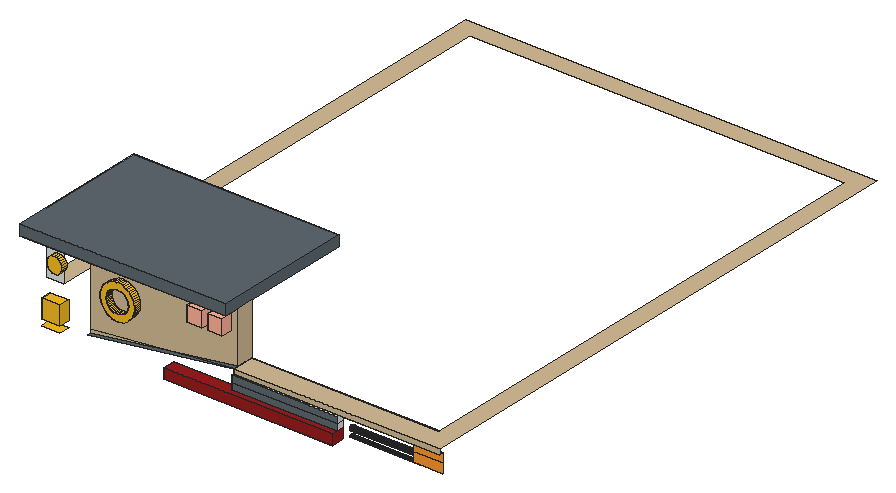
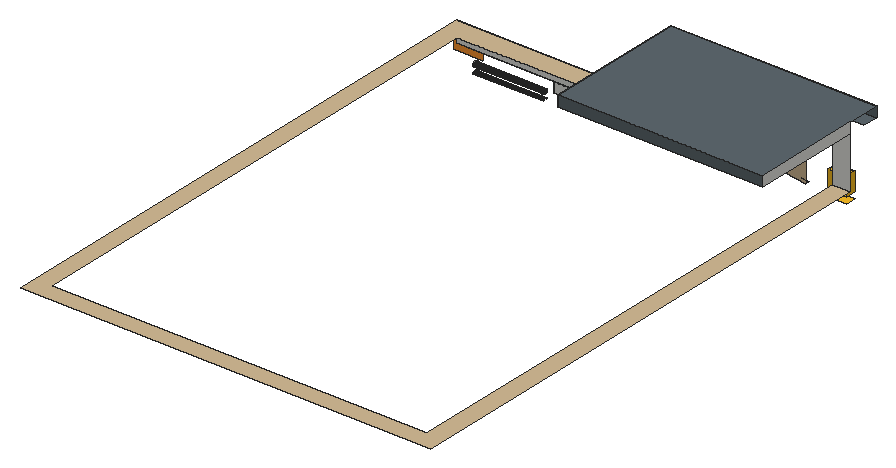
# SketchUp Ruby script. Lengths in inches.
U = 1.inch
M = Sketchup.active_model
def pt(a) = Geom::Point3d.new(a.map { |v| v * U })
def face(e, loops, mat)
  f = e.add_face(loops[0].map { |a| pt(a) })
  loops[1..].each { |l| e.add_face(l.map { |a| pt(a) }).erase! }
  f.material = f.back_material = mat if mat
  f
end
# faces: each face lists its corners as indices into pts; further lists are holes
def faces(e, pts, list, mat = nil) = list.each { |f| face(e, (f[0].is_a?(Array) ? f : [f]).map { |l| l.map { |i| pts[i] } }, mat) }
# xy, xz, yz: faces in a plane at the given z, y or x. An outline is a flat list of corners, or four numbers for a rectangle; further outlines are holes
def ring(l) = l.size == 4 ? [[l[0], l[1]], [l[2], l[1]], [l[2], l[3]], [l[0], l[3]]] : l.each_slice(2).to_a
def flat(e, list, mat, &to3) = list.each { |f| face(e, (f[0].is_a?(Array) ? f : [f]).map { |l| ring(l).map { |u, v| to3.(u, v) } }, mat) }
def xy(e, z, list, mat = nil) = flat(e, list, mat) { |x, y| [x, y, z] }
def xz(e, y, list, mat = nil) = flat(e, list, mat) { |x, z| [x, y, z] }
def yz(e, x, list, mat = nil) = flat(e, list, mat) { |y, z| [x, y, z] }
def lines(e, pts, list) = list.each { |a, b| e.add_line(pt(pts[a]), pt(pts[b])) }
# prism: a flat outline (further loops are holes) pulled along v
def prism(e, loops, v, mat = nil)
  f = face(e, loops, mat); d = Geom::Vector3d.new(v.map { |x| x * U })
  f.pushpull(f.normal.samedirection?(d) ? d.length : -d.length)
end
def box(e, o, s, mat = nil) = prism(e, [[o, [o[0] + s[0], o[1], o[2]], [o[0] + s[0], o[1] + s[1], o[2]], [o[0], o[1] + s[1], o[2]]]], [0, 0, s[2]], mat)
def at(x, y, z, deg = 0) = Geom::Transformation.translation(pt([x, y, z])) * Geom::Transformation.rotation(ORIGIN, Z_AXIS, deg.degrees)
def axes(o, x, y, z) = Geom::Transformation.new([*x, 0, *y, 0, *z, 0, *pt(o).to_a, 1])
def part(name) = M.definitions.add(name)
# library, detail: a bought-in or finely detailed component or shape, given as its bounding box
def library(name, o, s) = part(name).tap { |d| box(d.entities, o, s) }
def detail(e, o, s) = box(e.add_group.entities, o, s)
def put(e, d, t, mat = nil) = e.add_instance(d, t).tap { |i| i.material = mat if mat }
def group(e, t, mat = nil) = e.add_group.tap { |g| g.transformation = t; g.material = mat if mat }.entities
root = M.entities
M.materials.add("[0045_Goldenrod]").color = [249, 189, 36]
M.materials.add("[Color A04]").color = [155, 30, 30]
M.materials.add("[Color B02]").color = [255, 178, 153]
M.materials.add("[Color C04]").color = [255, 153, 50]
M.materials.add("[Formica Beige]").color = [211, 187, 149]
M.materials.add("[Formica Laminate Dark]").color = [50, 53, 60]
M.materials.add("[Formica Speckled Grey]").color = [94, 105, 111]
xy(root,310.29,[[175.33,79.24,383.64,94.74]],"[Color A04]")
xy(root,314.74,[[23.1,81.43,45.78,94.74]],"[0045_Goldenrod]")
xy(root,317.54,[[411.92,104.06,412.58,104.14,413.2,104.4,413.49,104.62,410.35,104.62,410.64,104.4,411.25,104.14],[410.35,104.62,413.49,104.62,413.73,104.81,414.14,105.34,414.39,105.95,414.48,106.62,414.39,107.28,414.14,107.9,413.73,108.43,413.2,108.84,412.58,109.09,411.92,109.18,411.25,109.09,410.64,108.84,410.11,108.43,409.7,107.9,409.44,107.28,409.36,106.62,409.44,105.95,409.7,105.34,410.11,104.81]])
xy(root,318.0625,[[440.11,104.06,440.77,104.14,441.39,104.4,441.92,104.81,442.32,105.34,442.58,105.95,442.67,106.62,442.58,107.28,442.32,107.9,441.92,108.43,441.39,108.84,440.77,109.09,440.11,109.18,439.44,109.09,438.82,108.84,438.29,108.43,437.89,107.9,437.63,107.28,437.54,106.62,437.63,105.95,437.89,105.34,438.29,104.81,438.82,104.4,439.44,104.14]])
xy(root,322.3,[[23.1,81.43,45.78,94.74]],"[0045_Goldenrod]")
xy(root,322.92,[[253.89,86.55,383.64,94.74]])
xy(root,322.92,[[175.33,79.24,383.64,79.24,383.64,86.55,253.89,86.55,253.89,94.74,175.33,94.74]],"[Color A04]")
xy(root,330.28,[[253.89,86.55,383.64,94.74]])
xy(root,338.91,[[253.89,86.55,383.64,89.43],[253.89,89.43,383.64,94.74],[253.89,94.74,383.64,116.19]])
xy(root,338.91,[[383.64,89.43,470.23,116.19],[470.23,89.43,506.36,94.74]],"[Formica Beige]")
xy(root,344.99,[[23.1,81.43,45.78,94.74]],"[0045_Goldenrod]")
xy(root,345.125,[[253.89,89.43,506.36,89.43,506.36,761.28,1.43,761.28,1.43,116.19,22.875,116.19,22.875,739.83,484.91,739.83,484.91,116.19,253.89,116.19]],"[Formica Beige]")
xy(root,381.62,[[202.13,81.55,220.38,94.74],[227.32,81.55,245.57,94.74]],"[Color B02]")
xy(root,399.87,[[202.13,81.55,220.38,94.74],[227.32,81.55,245.57,94.74]],"[Color B02]")
xy(root,408.81,[[1.43,76.18,73.65,94.74],[73.65,76.18,253.89,94.74],[1.43,116.19,253.89,250.25]],"[Formica Speckled Grey]")
xy(root,421.875,[[1.43,76.18,253.89,250.25]],"[Formica Speckled Grey]")
xz(root,76.18,[[1.43,408.81,253.89,421.875]],"[Formica Speckled Grey]")
xz(root,79.24,[[175.33,310.29,383.64,322.92]],"[Color A04]")
xz(root,81.43,[[23.1,322.3,45.78,344.99]],"[0045_Goldenrod]")
xz(root,81.55,[[202.13,381.62,220.38,399.87],[227.32,381.62,245.57,399.87]],"[Color B02]")
xz(root,85.93,[[[113.16,349,115.38,349.14,117.58,349.52,119.73,350.13,121.8,350.95,123.77,351.99,125.63,353.23,127.34,354.66,128.9,356.26,130.28,358.01,131.47,359.9,132.46,361.9,133.23,363.99,133.78,366.15,134.1,368.36,134.18,370.59,134.04,372.82,133.66,375.01,133.05,377.16,132.23,379.23,131.1875,381.21,129.95,383.0625,128.52,384.78,126.92,386.33,125.17,387.71,123.28,388.9,121.28,389.89,119.19,390.66,117.03,391.21,114.82,391.53,112.59,391.62,110.36,391.47,108.17,391.09,106.02,390.49,103.95,389.66,101.97,388.62,100.12,387.38,98.4,385.96,96.85,384.36,95.47,382.61,94.28,380.72,93.29,378.72,92.52,376.625,91.97,374.46,91.65,372.25,91.5625,370.03,91.71,367.8,92.09,365.6,92.69,363.45,93.52,361.38,94.56,359.41,95.8,357.55,97.23,355.84,98.82,354.28,100.58,352.9,102.46,351.71,104.46,350.72,106.56,349.95,108.72,349.4,110.93,349.08],[113.05,356.63,111.625,356.69,110.21,356.89,108.82,357.25,107.48,357.74,106.19,358.375,104.98,359.14,103.86,360.02,102.83,361.02,101.92,362.125,101.12,363.3125,100.46,364.58,99.92,365.91,99.54,367.29,99.29,368.7,99.2,370.125,99.26,371.56,99.46,372.97,99.8125,374.36,100.31,375.7,100.94,376.99,101.7,378.2,102.59,379.32,103.59,380.35,104.6875,381.26,105.88,382.06,107.15,382.73,108.48,383.26,109.85,383.65,111.26,383.89,112.69,383.98,114.12,383.93,115.54,383.72,116.93,383.37,118.27,382.875,119.55,382.24,120.76,381.48,121.89,380.59,122.91,379.59,123.83,378.49,124.625,377.3,125.29,376.03,125.82,374.71,126.21,373.33,126.45,371.92,126.55,370.49,126.49,369.06,126.29,367.64,125.93,366.25,125.4375,364.91,124.81,363.63,124.04,362.42,123.16,361.29,122.16,360.27,121.06,359.35,119.87,358.56,118.6,357.89,117.27,357.36,115.89,356.97,114.48,356.73]]],"[0045_Goldenrod]")
xz(root,86.55,[[253.89,322.92,383.64,330.28],[253.89,330.28,383.64,338.91]],"[Formica Speckled Grey]")
xz(root,87.62,[[34.11,372.72,36.6,373.05,38.92,374.01,40.92,375.54,42.45,377.53,43.41,379.85,43.74,382.34,43.41,384.83,42.45,387.15,40.92,389.15,38.92,390.68,36.6,391.64,34.11,391.97,31.62,391.64,29.3,390.68,27.3,389.15,25.78,387.15,24.8125,384.83,24.49,382.34,24.8125,379.85,25.78,377.53,27.3,375.54,29.3,374.01,31.62,373.05]],"[0045_Goldenrod]")
xz(root,89.43,[[253.89,338.91,506.36,345.125]],"[Formica Beige]")
xz(root,94.74,[[175.33,310.29,383.64,322.92],[253.89,322.92,383.64,330.28],[253.89,330.28,383.64,338.91],[202.13,381.62,220.38,399.87],[227.32,381.62,245.57,399.87]])
xz(root,94.74,[[470.23,315.65,506.36,327.28],[470.23,327.28,506.36,338.91]],"[Color C04]")
xz(root,94.74,[[[73.65,318.75,253.89,345.125,253.89,408.81,73.65,408.81],[113.16,349,110.93,349.08,108.72,349.4,106.56,349.95,104.46,350.72,102.46,351.71,100.58,352.9,98.82,354.28,97.23,355.84,95.8,357.55,94.56,359.41,93.52,361.38,92.69,363.45,92.09,365.6,91.71,367.8,91.5625,370.03,91.65,372.25,91.97,374.46,92.52,376.625,93.29,378.72,94.28,380.72,95.47,382.61,96.85,384.36,98.4,385.96,100.12,387.38,101.97,388.62,103.95,389.66,106.02,390.49,108.17,391.09,110.36,391.47,112.59,391.62,114.82,391.53,117.03,391.21,119.19,390.66,121.28,389.89,123.28,388.9,125.17,387.71,126.92,386.33,128.52,384.78,129.95,383.0625,131.1875,381.21,132.23,379.23,133.05,377.16,133.66,375.01,134.04,372.82,134.18,370.59,134.1,368.36,133.78,366.15,133.23,363.99,132.46,361.9,131.47,359.9,130.28,358.01,128.9,356.26,127.34,354.66,125.63,353.23,123.77,351.99,121.8,350.95,119.73,350.13,117.58,349.52,115.38,349.14],[202.13,381.62,220.38,399.87],[227.32,381.62,245.57,399.87]],[113.05,356.63,114.48,356.73,115.89,356.97,117.27,357.36,118.6,357.89,119.87,358.56,121.06,359.35,122.16,360.27,123.16,361.29,124.04,362.42,124.81,363.63,125.4375,364.91,125.93,366.25,126.29,367.64,126.49,369.06,126.55,370.49,126.45,371.92,126.21,373.33,125.82,374.71,125.29,376.03,124.625,377.3,123.83,378.49,122.91,379.59,121.89,380.59,120.76,381.48,119.55,382.24,118.27,382.875,116.93,383.37,115.54,383.72,114.12,383.93,112.69,383.98,111.26,383.89,109.85,383.65,108.48,383.26,107.15,382.73,105.88,382.06,104.6875,381.26,103.59,380.35,102.59,379.32,101.7,378.2,100.94,376.99,100.31,375.7,99.8125,374.36,99.46,372.97,99.26,371.56,99.2,370.125,99.29,368.7,99.54,367.29,99.92,365.91,100.46,364.58,101.12,363.3125,101.92,362.125,102.83,361.02,103.86,360.02,104.98,359.14,106.19,358.375,107.48,357.74,108.82,357.25,110.21,356.89,111.625,356.69]],"[Formica Beige]")
xz(root,116.19,[[253.89,338.91,484.91,345.125],[1.43,345.125,22.875,408.81]])
xz(root,250.25,[[1.43,408.81,253.89,421.875]],"[Formica Speckled Grey]")
yz(root,1.43,[[116.19,408.81,250.25,421.875]])
yz(root,23.1,[[81.43,322.3,94.74,344.99]],"[0045_Goldenrod]")
yz(root,45.78,[[81.43,322.3,94.74,344.99]],"[0045_Goldenrod]")
yz(root,175.33,[[79.24,310.29,94.74,322.92]],"[Color A04]")
yz(root,202.13,[[81.55,381.62,94.74,399.87]],"[Color B02]")
yz(root,220.38,[[81.55,381.62,94.74,399.87]],"[Color B02]")
yz(root,227.32,[[81.55,381.62,94.74,399.87]],"[Color B02]")
yz(root,245.57,[[81.55,381.62,94.74,399.87]],"[Color B02]")
yz(root,253.89,[[86.55,322.92,94.74,330.28],[86.55,330.28,94.74,338.91],[89.43,338.91,116.19,345.125]])
yz(root,253.89,[[94.74,345.125,116.19,408.81]],"[Formica Beige]")
yz(root,253.89,[[76.18,408.81,250.25,421.875]],"[Formica Speckled Grey]")
yz(root,383.64,[[86.55,322.92,94.74,330.28],[86.55,330.28,94.74,338.91]])
yz(root,383.64,[[79.24,310.29,94.74,322.92]],"[Color A04]")
yz(root,470.23,[[107.5,314.66,108.24,314.76,108.93,315.05,109.53,315.51,109.99,316.1,110.27,316.79,110.37,317.54,110.27,318.28,109.99,318.98,109.53,319.57,108.93,320.03,108.24,320.32,107.5,320.41,106.75,320.32,106.06,320.03,105.46,319.57,105.01,318.98,104.72,318.28,104.62,317.54,104.72,316.79,105.01,316.1,105.46,315.51,106.06,315.05,106.75,314.76]])
p = [[470.23,104.72,308.09],[470.23,105.01,308.79],[383.64,105.01,308.79],[383.64,104.72,308.09],[470.23,109.99,308.79],[470.23,110.27,308.09],
  [383.64,110.27,308.09],[383.64,109.99,308.79],[470.23,105.46,309.38],[383.64,105.46,309.38],[470.23,109.53,309.38],[383.64,109.53,309.38],
  [470.23,106.06,309.84],[383.64,106.06,309.84],[470.23,108.93,309.84],[383.64,108.93,309.84],[470.23,106.75,310.13],[383.64,106.75,310.13],
  [470.23,108.24,310.13],[383.64,108.24,310.13],[470.23,107.5,310.23],[383.64,107.5,310.23],[470.23,107.5,314.66],[470.23,106.75,314.76],
  [383.64,106.75,314.76],[383.64,107.5,314.66],[470.23,108.24,314.76],[383.64,108.24,314.76],[470.23,106.06,315.05],[383.64,106.06,315.05],
  [470.23,108.93,315.05],[383.64,108.93,315.05],[470.23,105.46,315.51],[383.64,105.46,315.51],[470.23,109.53,315.51],[383.64,109.53,315.51],
  [470.23,105.01,316.1],[383.64,105.01,316.1],[470.23,109.99,316.1],[383.64,109.99,316.1],[470.23,104.72,316.79],[383.64,104.72,316.79],
  [470.23,110.27,316.79],[383.64,110.27,316.79],[470.23,104.62,317.54],[413.49,104.62,317.54],[410.35,104.62,317.54],[383.64,104.62,317.54],
  [470.23,110.37,317.54],[383.64,110.37,317.54],[470.23,104.72,318.28],[383.64,104.72,318.28],[470.23,110.27,318.28],[383.64,110.27,318.28],
  [470.23,105.01,318.98],[383.64,105.01,318.98],[470.23,109.99,318.98],[383.64,109.99,318.98],[253.89,94.74,345.125],[73.65,94.74,318.75],
  [73.65,89.43,318.75],[253.89,89.43,345.125],[470.23,105.46,319.57],[383.64,105.46,319.57],[470.23,109.53,319.57],[383.64,109.53,319.57],
  [470.23,106.06,320.03],[383.64,106.06,320.03],[470.23,108.93,320.03],[383.64,108.93,320.03],[470.23,106.75,320.32],[383.64,106.75,320.32],
  [470.23,108.24,320.32],[383.64,108.24,320.32],[470.23,107.5,320.41],[383.64,107.5,320.41],[110.93,94.74,349.08],[113.16,94.74,349],
  [113.16,85.93,349],[110.93,85.93,349.08],[115.38,94.74,349.14],[115.38,85.93,349.14],[108.72,94.74,349.4],[108.72,85.93,349.4],
  [117.58,94.74,349.52],[117.58,85.93,349.52],[106.56,94.74,349.95],[106.56,85.93,349.95],[119.73,94.74,350.13],[119.73,85.93,350.13],
  [104.46,94.74,350.72],[104.46,85.93,350.72],[121.8,94.74,350.95],[121.8,85.93,350.95],[102.46,94.74,351.71],[102.46,85.93,351.71],
  [123.77,94.74,351.99],[123.77,85.93,351.99],[100.58,94.74,352.9],[100.58,85.93,352.9],[125.63,94.74,353.23],[125.63,85.93,353.23],
  [98.82,94.74,354.28],[98.82,85.93,354.28],[127.34,94.74,354.66],[127.34,85.93,354.66],[97.23,94.74,355.84],[97.23,85.93,355.84],
  [128.9,94.74,356.26],[128.9,85.93,356.26],[95.8,94.74,357.55],[95.8,85.93,357.55],[130.28,94.74,358.01],[130.28,85.93,358.01],
  [113.05,94.74,356.63],[111.625,94.74,356.69],[111.625,85.93,356.69],[113.05,85.93,356.63],[114.48,94.74,356.73],[114.48,85.93,356.73],
  [110.21,94.74,356.89],[110.21,85.93,356.89],[115.89,94.74,356.97],[115.89,85.93,356.97],[108.82,94.74,357.25],[108.82,85.93,357.25],
  [117.27,94.74,357.36],[117.27,85.93,357.36],[107.48,94.74,357.74],[107.48,85.93,357.74],[118.6,94.74,357.89],[118.6,85.93,357.89],
  [94.56,94.74,359.41],[94.56,85.93,359.41],[106.19,94.74,358.375],[106.19,85.93,358.375],[119.87,94.74,358.56],[119.87,85.93,358.56],
  [131.47,94.74,359.9],[131.47,85.93,359.9],[104.98,94.74,359.14],[104.98,85.93,359.14],[121.06,94.74,359.35],[121.06,85.93,359.35],
  [103.86,94.74,360.02],[103.86,85.93,360.02],[93.52,94.74,361.38],[93.52,85.93,361.38],[122.16,94.74,360.27],[122.16,85.93,360.27],
  [132.46,94.74,361.9],[132.46,85.93,361.9],[102.83,94.74,361.02],[102.83,85.93,361.02],[123.16,94.74,361.29],[123.16,85.93,361.29],
  [101.92,94.74,362.125],[101.92,85.93,362.125],[124.04,94.74,362.42],[124.04,85.93,362.42],[92.69,94.74,363.45],[92.69,85.93,363.45],
  [133.23,94.74,363.99],[133.23,85.93,363.99],[101.12,94.74,363.3125],[101.12,85.93,363.3125],[124.81,94.74,363.63],[124.81,85.93,363.63],
  [100.46,94.74,364.58],[100.46,85.93,364.58],[92.09,94.74,365.6],[92.09,85.93,365.6],[125.4375,94.74,364.91],[125.4375,85.93,364.91],
  [133.78,94.74,366.15],[133.78,85.93,366.15],[99.92,94.74,365.91],[99.92,85.93,365.91],[125.93,94.74,366.25],[125.93,85.93,366.25],
  [91.71,94.74,367.8],[91.71,85.93,367.8],[99.54,94.74,367.29],[99.54,85.93,367.29],[134.1,94.74,368.36],[134.1,85.93,368.36],
  [126.29,94.74,367.64],[126.29,85.93,367.64],[99.29,94.74,368.7],[99.29,85.93,368.7],[126.49,94.74,369.06],[126.49,85.93,369.06],
  [91.5625,94.74,370.03],[91.5625,85.93,370.03],[134.18,94.74,370.59],[134.18,85.93,370.59],[99.2,94.74,370.125],[99.2,85.93,370.125],
  [126.55,94.74,370.49],[126.55,85.93,370.49],[91.65,94.74,372.25],[91.65,85.93,372.25],[99.26,94.74,371.56],[99.26,85.93,371.56],
  [126.45,94.74,371.92],[126.45,85.93,371.92],[134.04,94.74,372.82],[134.04,85.93,372.82],[99.46,94.74,372.97],[99.46,85.93,372.97],
  [126.21,94.74,373.33],[126.21,85.93,373.33],[91.97,94.74,374.46],[91.97,85.93,374.46],[31.62,94.74,373.05],[34.11,94.74,372.72],
  [34.11,87.62,372.72],[31.62,87.62,373.05],[36.6,94.74,373.05],[36.6,87.62,373.05],[133.66,94.74,375.01],[133.66,85.93,375.01],
  [99.8125,94.74,374.36],[99.8125,85.93,374.36],[29.3,94.74,374.01],[29.3,87.62,374.01],[38.92,94.74,374.01],[38.92,87.62,374.01],
  [125.82,94.74,374.71],[125.82,85.93,374.71],[27.3,94.74,375.54],[27.3,87.62,375.54],[40.92,94.74,375.54],[40.92,87.62,375.54],
  [100.31,94.74,375.7],[100.31,85.93,375.7],[92.52,94.74,376.625],[92.52,85.93,376.625],[125.29,94.74,376.03],[125.29,85.93,376.03],
  [133.05,94.74,377.16],[133.05,85.93,377.16],[25.78,94.74,377.53],[25.78,87.62,377.53],[42.45,94.74,377.53],[42.45,87.62,377.53],
  [100.94,94.74,376.99],[100.94,85.93,376.99],[124.625,94.74,377.3],[124.625,85.93,377.3],[93.29,94.74,378.72],[93.29,85.93,378.72],
  [101.7,94.74,378.2],[101.7,85.93,378.2],[132.23,94.74,379.23],[132.23,85.93,379.23],[123.83,94.74,378.49],[123.83,85.93,378.49],
  [24.8125,94.74,379.85],[24.8125,87.62,379.85],[43.41,94.74,379.85],[43.41,87.62,379.85],[102.59,94.74,379.32],[102.59,85.93,379.32],
  [122.91,94.74,379.59],[122.91,85.93,379.59],[94.28,94.74,380.72],[94.28,85.93,380.72],[131.1875,94.74,381.21],[131.1875,85.93,381.21],
  [103.59,94.74,380.35],[103.59,85.93,380.35],[121.89,94.74,380.59],[121.89,85.93,380.59],[24.49,94.74,382.34],[24.49,87.62,382.34],
  [43.74,94.74,382.34],[43.74,87.62,382.34],[104.6875,94.74,381.26],[104.6875,85.93,381.26],[120.76,94.74,381.48],[120.76,85.93,381.48],
  [95.47,94.74,382.61],[95.47,85.93,382.61],[129.95,94.74,383.0625],[129.95,85.93,383.0625],[105.88,94.74,382.06],[105.88,85.93,382.06],
  [119.55,94.74,382.24],[119.55,85.93,382.24],[107.15,94.74,382.73],[107.15,85.93,382.73],[118.27,94.74,382.875],[118.27,85.93,382.875],
  [24.8125,94.74,384.83],[24.8125,87.62,384.83],[43.41,94.74,384.83],[43.41,87.62,384.83],[96.85,94.74,384.36],[96.85,85.93,384.36],
  [108.48,94.74,383.26],[108.48,85.93,383.26],[116.93,94.74,383.37],[116.93,85.93,383.37],[128.52,94.74,384.78],[128.52,85.93,384.78],
  [109.85,94.74,383.65],[109.85,85.93,383.65],[115.54,94.74,383.72],[115.54,85.93,383.72],[111.26,94.74,383.89],[111.26,85.93,383.89],
  [114.12,94.74,383.93],[114.12,85.93,383.93],[112.69,94.74,383.98],[112.69,85.93,383.98],[98.4,94.74,385.96],[98.4,85.93,385.96],
  [126.92,94.74,386.33],[126.92,85.93,386.33],[25.78,94.74,387.15],[25.78,87.62,387.15],[42.45,94.74,387.15],[42.45,87.62,387.15],
  [100.12,94.74,387.38],[100.12,85.93,387.38],[125.17,94.74,387.71],[125.17,85.93,387.71],[27.3,94.74,389.15],[27.3,87.62,389.15],
  [40.92,94.74,389.15],[40.92,87.62,389.15],[101.97,94.74,388.62],[101.97,85.93,388.62],[123.28,94.74,388.9],[123.28,85.93,388.9],
  [103.95,94.74,389.66],[103.95,85.93,389.66],[121.28,94.74,389.89],[121.28,85.93,389.89],[29.3,94.74,390.68],[29.3,87.62,390.68],
  [38.92,94.74,390.68],[38.92,87.62,390.68],[106.02,94.74,390.49],[106.02,85.93,390.49],[119.19,94.74,390.66],[119.19,85.93,390.66],
  [108.17,94.74,391.09],[108.17,85.93,391.09],[117.03,94.74,391.21],[117.03,85.93,391.21],[31.62,94.74,391.64],[31.62,87.62,391.64],
  [36.6,94.74,391.64],[36.6,87.62,391.64],[110.36,94.74,391.47],[110.36,85.93,391.47],[114.82,94.74,391.53],[114.82,85.93,391.53],
  [112.59,94.74,391.62],[112.59,85.93,391.62],[34.11,94.74,391.97],[34.11,87.62,391.97],[73.65,94.74,322.92]]
faces(root,p,[[0,1,2,3],[4,5,6,7],[1,8,9,2],[10,4,7,11],[8,12,13,9],[14,10,11,15],[12,16,17,13],[18,14,15,19],
  [16,20,21,17],[20,18,19,21],[22,23,24,25],[26,22,25,27],[23,28,29,24],[30,26,27,31],[28,32,33,29],[34,30,31,35],
  [32,36,37,33],[38,34,35,39],[36,40,41,37],[42,38,39,43],[40,44,45,46,47,41],[48,42,43,49],[44,50,51,47,46,45],[52,48,49,53],
  [50,54,55,51],[56,52,53,57],[54,62,63,55],[64,56,57,65],[62,66,67,63],[68,64,65,69],[66,70,71,67],[72,68,69,73],
  [70,74,75,71],[74,72,73,75]],"[Formica Laminate Dark]")
faces(root,p,[[58,59,60,61]],"[Formica Speckled Grey]")
faces(root,p,[[76,77,78,79],[77,80,81,78],[82,76,79,83],[80,84,85,81],[86,82,83,87],[84,88,89,85],[90,86,87,91],[88,92,93,89],
  [94,90,91,95],[92,96,97,93],[98,94,95,99],[96,100,101,97],[102,98,99,103],[100,104,105,101],[106,102,103,107],[104,108,109,105],
  [110,106,107,111],[108,112,113,109],[114,115,116,117],[118,114,117,119],[115,120,121,116],[122,118,119,123],[120,124,125,121],[126,122,123,127],
  [124,128,129,125],[130,126,127,131],[132,110,111,133],[128,134,135,129],[136,130,131,137],[112,138,139,113],[134,140,141,135],[142,136,137,143],
  [140,144,145,141],[146,132,133,147],[148,142,143,149],[138,150,151,139],[144,152,153,145],[154,148,149,155],[152,156,157,153],[158,154,155,159],
  [160,146,147,161],[150,162,163,151],[156,164,165,157],[166,158,159,167],[164,168,169,165],[170,160,161,171],[172,166,167,173],[162,174,175,163],
  [168,176,177,169],[178,172,173,179],[180,170,171,181],[176,182,183,177],[174,184,185,175],[186,178,179,187],[182,188,189,183],[190,186,187,191],
  [192,180,181,193],[184,194,195,185],[188,196,197,189],[198,190,191,199],[200,192,193,201],[196,202,203,197],[204,198,199,205],[194,206,207,195],
  [202,208,209,203],[210,204,205,211],[212,200,201,213],[214,215,216,217],[215,218,219,216],[206,220,221,207],[208,222,223,209],[224,214,217,225],
  [218,226,227,219],[228,210,211,229],[230,224,225,231],[226,232,233,227],[222,234,235,223],[236,212,213,237],[238,228,229,239],[220,240,241,221],
  [242,230,231,243],[232,244,245,233],[234,246,247,235],[248,238,239,249],[250,236,237,251],[246,252,253,247],[240,254,255,241],[256,248,249,257],
  [258,242,243,259],[244,260,261,245],[252,262,263,253],[264,256,257,265],[266,250,251,267],[254,268,269,255],[262,270,271,263],[272,264,265,273],
  [274,258,259,275],[260,276,277,261],[270,278,279,271],[280,272,273,281],[282,266,267,283],[268,284,285,269],[278,286,287,279],[288,280,281,289],
  [286,290,291,287],[292,288,289,293],[294,274,275,295],[276,296,297,277],[298,282,283,299],[290,300,301,291],[302,292,293,303],[284,304,305,285],
  [300,306,307,301],[308,302,303,309],[306,310,311,307],[312,308,309,313],[310,314,315,311],[314,312,313,315],[316,298,299,317],[304,318,319,305],
  [320,294,295,321],[296,322,323,297],[324,316,317,325],[318,326,327,319],[328,320,321,329],[322,330,331,323],[332,324,325,333],[326,334,335,327],
  [336,332,333,337],[334,338,339,335],[340,328,329,341],[330,342,343,331],[344,336,337,345],[338,346,347,339],[348,344,345,349],[346,350,351,347],
  [352,340,341,353],[342,354,355,343],[356,348,349,357],[350,358,359,351],[360,356,357,361],[358,360,361,359],[362,352,353,363],[354,362,363,355]],"[0045_Goldenrod]")
lines(root,p,[[364,61]])
